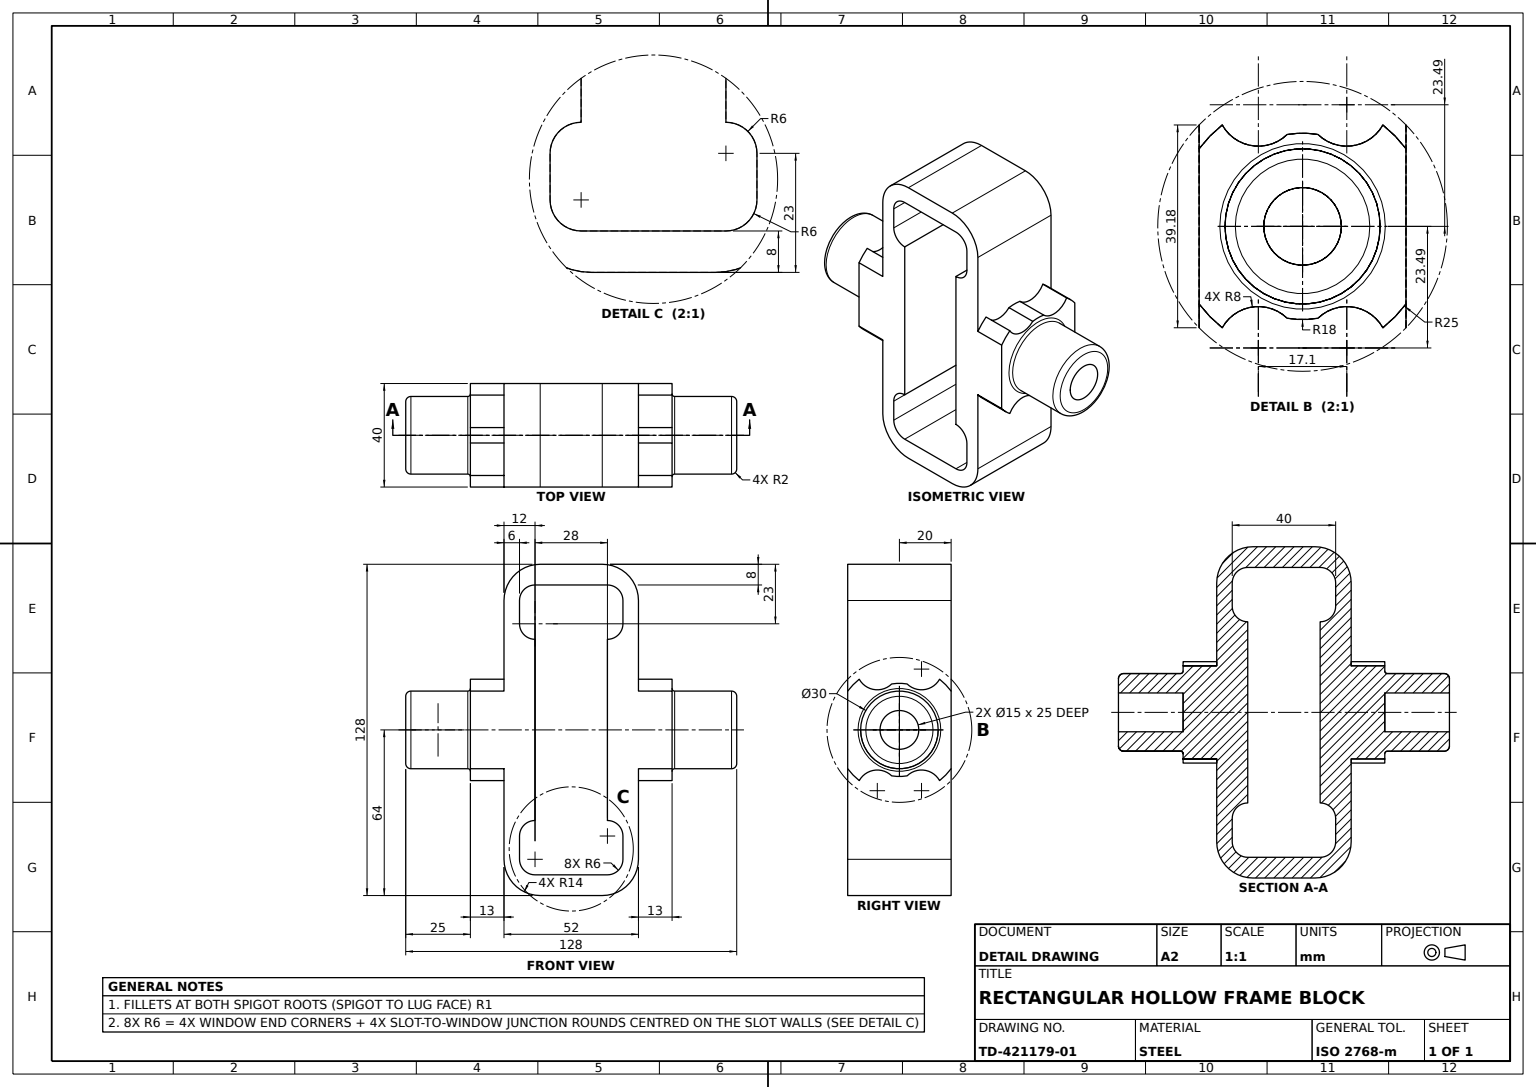
solid
v1 (-64,0,27.5)
v2 (-64,0,12.5)
e1 v1 v2 CIRCLE(AX(P(-64,0,20),D(-1,0,0),D(0,0,1)),7.5)
e2 v2 v1 CIRCLE(AX(P(-64,0,20),D(-1,0,0),D(0,0,1)),7.5)
v3 (-64,0,7)
v4 (-64,0,33)
e3 v3 v4 CIRCLE(AX(P(-64,0,20),D(-1,0,0),D(0,0,1)),13)
e4 v4 v3 CIRCLE(AX(P(-64,0,20),D(-1,0,0),D(0,0,1)),13)
face PLANE(AX(P(-64,0,20),D(-1,0,0),D(0,0,1))) [-e1 -e2] [e3 e4]
v5 (39,-15,40)
v6 (26,-15,40)
e5 v5 v6 LINE
v7 (39,15,40)
e6 v7 v5 LINE
v8 (26,15,40)
e7 v7 v8 LINE
v9 (26,50,40)
e8 v8 v9 LINE
v10 (12,64,40)
e9 v9 v10 CIRCLE(AX(P(12,50,40),D(0,0,1),D(-1,0,0)),14)
v11 (-12,64,40)
e10 v10 v11 LINE
v12 (-26,50,40)
e11 v11 v12 CIRCLE(AX(P(-12,50,40),D(0,0,1),D(-1,0,0)),14)
v13 (-26,15,40)
e12 v12 v13 LINE
v14 (-39,15,40)
e13 v14 v13 LINE
v15 (-39,-15,40)
e14 v15 v14 LINE
v16 (-26,-15,40)
e15 v15 v16 LINE
v17 (-26,-50,40)
e16 v16 v17 LINE
v18 (-12,-64,40)
e17 v17 v18 CIRCLE(AX(P(-12,-50,40),D(0,0,1),D(-1,0,0)),14)
v19 (12,-64,40)
e18 v18 v19 LINE
v20 (26,-50,40)
e19 v19 v20 CIRCLE(AX(P(12,-50,40),D(0,0,1),D(-1,0,0)),14)
e20 v20 v6 LINE
v21 (14,-35,40)
v22 (14,35,40)
e21 v21 v22 LINE
v23 (20,-41,40)
e22 v23 v21 CIRCLE(AX(P(14,-41,40),D(0,0,1),D(-1,0,0)),6)
v24 (20,-50,40)
e23 v24 v23 LINE
v25 (14,-56,40)
e24 v25 v24 CIRCLE(AX(P(14,-50,40),D(0,0,1),D(-1,0,0)),6)
v26 (-14,-56,40)
e25 v26 v25 LINE
v27 (-20,-50,40)
e26 v27 v26 CIRCLE(AX(P(-14,-50,40),D(0,0,1),D(-1,0,0)),6)
v28 (-20,-41,40)
e27 v28 v27 LINE
v29 (-14,-35,40)
e28 v29 v28 CIRCLE(AX(P(-14,-41,40),D(0,0,1),D(-1,0,0)),6)
v30 (-14,35,40)
e29 v30 v29 LINE
v31 (-20,41,40)
e30 v31 v30 CIRCLE(AX(P(-14,41,40),D(0,0,1),D(1,0,0)),6)
v32 (-20,50,40)
e31 v32 v31 LINE
v33 (-14,56,40)
e32 v33 v32 CIRCLE(AX(P(-14,50,40),D(0,0,1),D(-1,0,0)),6)
v34 (14,56,40)
e33 v34 v33 LINE
v35 (20,50,40)
e34 v35 v34 CIRCLE(AX(P(14,50,40),D(0,0,1),D(1,0,0)),6)
v36 (20,41,40)
e35 v36 v35 LINE
e36 v22 v36 CIRCLE(AX(P(14,41,40),D(0,0,1),D(-1,0,0)),6)
face PLANE(AX(P(12,-50,40),D(0,0,-1),D(-1,0,0))) rev [-e5 -e6 e7 e8 e9 e10 e11 e12 -e13 -e14 e15 e16 e17 e18 e19 e20] [-e21 -e22 -e23 -e24 -e25 -e26 -e27 -e28 -e29 -e30 -e31 -e32 -e33 -e34 -e35 -e36]
v37 (20,50,0)
e37 v37 v35 LINE
v38 (20,41,0)
e38 v38 v37 LINE
e39 v38 v36 LINE
face PLANE(AX(P(20,41,0),D(1,0,0),D(0,0,-1))) rev [e35 -e37 -e38 e39]
v39 (40,0,35)
v40 (39,0,36)
e40 v39 v40 CIRCLE(AX(P(40,0,36),D(0,1,0),D(0,0,1)),1)
v41 (40,0,5)
e41 v41 v39 CIRCLE(AX(P(40,0,20),D(1,0,0),D(0,0,-1)),15)
v42 (39,0,4)
e42 v41 v42 CIRCLE(AX(P(40,0,4),D(0,-1,0),D(0,0,-1)),1)
e43 v40 v42 CIRCLE(AX(P(39,0,20),D(-1,0,0),D(0,0,-1)),16)
face TORUS(AX(P(40,0,20),D(1,0,0),D(0,0,-1)),16,1) rev [-e40 -e41 e42 -e43]
v43 (-39,-15,0)
v44 (-26,-15,0)
e44 v43 v44 LINE
v45 (-26,-19.588598,4.46659)
e45 v44 v45 CIRCLE(AX(P(-26,0,20),D(-1,0,0),D(0,0,1)),25)
v46 (-39,-19.588598,4.46659)
e46 v46 v45 LINE
e47 v43 v46 CIRCLE(AX(P(-39,0,20),D(-1,0,0),D(0,0,1)),25)
face CYL(AX(P(-39,0,20),D(1,0,0),D(0,0,-1)),25) [e44 e45 -e46 -e47]
v47 (-14,35,0)
e48 v47 v30 LINE
v48 (-20,41,0)
e49 v48 v47 CIRCLE(AX(P(-14,41,0),D(0,0,1),D(1,0,0)),6)
e50 v48 v31 LINE
face CYL(AX(P(-14,41,0),D(0,0,1),D(1,0,0)),6) rev [-e48 -e49 e50 e30]
v49 (-14,56,0)
e51 v49 v33 LINE
v50 (-20,50,0)
e52 v50 v32 LINE
e53 v49 v50 CIRCLE(AX(P(-14,50,0),D(0,0,1),D(-1,0,0)),6)
face CYL(AX(P(-14,50,0),D(0,0,1),D(1,0,0)),6) rev [e51 e32 -e52 -e53]
v51 (39,-17.751859,17.021494)
v52 (39,-19.588598,4.46659)
e54 v51 v52 CIRCLE(AX(P(39,-23.492316,11.449496),D(-1,0,0),D(0,0,-1)),8)
v53 (26,-17.751859,17.021494)
e55 v51 v53 LINE
v54 (26,-19.588598,4.46659)
e56 v53 v54 CIRCLE(AX(P(26,-23.492316,11.449496),D(-1,0,0),D(0,0,-1)),8)
e57 v52 v54 LINE
face CYL(AX(P(39,-23.492316,11.449496),D(-1,0,0),D(0,0,1)),8) rev [-e54 e55 e56 -e57]
v55 (-39,17.751859,22.978506)
v56 (-26,17.751859,22.978506)
e58 v55 v56 LINE
v57 (-39,19.588598,35.53341)
e59 v57 v55 CIRCLE(AX(P(-39,23.492316,28.550504),D(1,0,0),D(0,0,1)),8)
v58 (-26,19.588598,35.53341)
e60 v57 v58 LINE
e61 v58 v56 CIRCLE(AX(P(-26,23.492316,28.550504),D(1,0,0),D(0,0,1)),8)
face CYL(AX(P(-39,23.492316,28.550504),D(1,0,0),D(0,0,-1)),8) rev [-e58 -e59 e60 e61]
e62 v42 v40 CIRCLE(AX(P(39,0,20),D(-1,0,0),D(0,0,-1)),16)
e63 v39 v41 CIRCLE(AX(P(40,0,20),D(1,0,0),D(0,0,-1)),15)
face TORUS(AX(P(40,0,20),D(1,0,0),D(0,0,-1)),16,1) rev [e40 -e62 -e42 -e63]
v59 (26,50,0)
e64 v9 v59 LINE
v60 (12,64,0)
e65 v59 v60 CIRCLE(AX(P(12,50,0),D(0,0,1),D(-1,0,0)),14)
e66 v10 v60 LINE
face CYL(AX(P(12,50,40),D(0,0,-1),D(-1,0,0)),14) [-e9 e64 e65 -e66]
v61 (39,-17.751859,22.978506)
v62 (26,-17.751859,22.978506)
e67 v61 v62 LINE
v63 (39,-19.588598,35.53341)
e68 v63 v61 CIRCLE(AX(P(39,-23.492316,28.550504),D(-1,0,0),D(0,0,-1)),8)
v64 (26,-19.588598,35.53341)
e69 v63 v64 LINE
e70 v64 v62 CIRCLE(AX(P(26,-23.492316,28.550504),D(-1,0,0),D(0,0,-1)),8)
face CYL(AX(P(39,-23.492316,28.550504),D(-1,0,0),D(0,0,1)),8) rev [-e67 -e68 e69 e70]
v65 (-40,0,35)
v66 (-40,0,5)
e71 v65 v66 CIRCLE(AX(P(-40,0,20),D(-1,0,0),D(0,0,1)),15)
v67 (-62,0,5)
e72 v67 v66 LINE
v68 (-62,0,35)
e73 v67 v68 CIRCLE(AX(P(-62,0,20),D(1,0,0),D(0,0,1)),15)
e74 v68 v65 LINE
face CYL(AX(P(-64,0,20),D(1,0,0),D(0,0,-1)),15) [e71 -e72 e73 e74]
v69 (12,-64,0)
e75 v19 v69 LINE
v70 (26,-50,0)
e76 v69 v70 CIRCLE(AX(P(12,-50,0),D(0,0,1),D(-1,0,0)),14)
e77 v20 v70 LINE
face CYL(AX(P(12,-50,40),D(0,0,-1),D(-1,0,0)),14) [e75 e76 -e77 -e19]
v71 (-12,-64,0)
e78 v18 v71 LINE
v72 (-26,-50,0)
e79 v17 v72 LINE
e80 v72 v71 CIRCLE(AX(P(-12,-50,0),D(0,0,1),D(-1,0,0)),14)
face CYL(AX(P(-12,-50,40),D(0,0,-1),D(-1,0,0)),14) [-e78 -e17 e79 e80]
v73 (39,19.588598,4.46659)
v74 (39,17.751859,17.021494)
e81 v73 v74 CIRCLE(AX(P(39,23.492316,11.449496),D(-1,0,0),D(0,0,-1)),8)
v75 (26,19.588598,4.46659)
e82 v73 v75 LINE
v76 (26,17.751859,17.021494)
e83 v75 v76 CIRCLE(AX(P(26,23.492316,11.449496),D(-1,0,0),D(0,0,-1)),8)
e84 v74 v76 LINE
face CYL(AX(P(39,23.492316,11.449496),D(-1,0,0),D(0,0,1)),8) rev [-e81 e82 e83 -e84]
v77 (26,-15,0)
e85 v54 v77 CIRCLE(AX(P(26,0,20),D(1,0,0),D(0,0,-1)),25)
v78 (39,-15,0)
e86 v78 v77 LINE
e87 v52 v78 CIRCLE(AX(P(39,0,20),D(1,0,0),D(0,0,-1)),25)
face CYL(AX(P(39,0,20),D(-1,0,0),D(0,0,1)),25) [e85 -e86 -e87 e57]
e88 v68 v4 CIRCLE(AX(P(-62,0,33),D(0,-1,0),D(0,0,-1)),2)
e89 v67 v3 CIRCLE(AX(P(-62,0,7),D(0,1,0),D(0,0,1)),2)
face TORUS(AX(P(-62,0,20),D(-1,0,0),D(0,0,1)),13,2) [-e4 -e88 -e73 e89]
e90 v62 v53 CIRCLE(AX(P(26,0,20),D(1,0,0),D(0,0,-1)),18)
e91 v61 v51 CIRCLE(AX(P(39,0,20),D(1,0,0),D(0,0,-1)),18)
face CYL(AX(P(39,0,20),D(-1,0,0),D(0,0,1)),18) [e67 e90 -e55 -e91]
e92 v5 v63 CIRCLE(AX(P(39,0,20),D(1,0,0),D(0,0,-1)),25)
e93 v6 v64 CIRCLE(AX(P(26,0,20),D(1,0,0),D(0,0,-1)),25)
face CYL(AX(P(39,0,20),D(-1,0,0),D(0,0,1)),25) [-e69 -e92 e5 e93]
v79 (-39,0,12.5)
e94 v2 v79 LINE
v80 (-39,0,27.5)
e95 v79 v80 CIRCLE(AX(P(-39,0,20),D(1,0,0),D(0,0,1)),7.5)
e96 v1 v80 LINE
face CYL(AX(P(-64,0,20),D(1,0,0),D(0,0,-1)),7.5) rev [e1 e94 e95 -e96]
v81 (-39,-17.751859,22.978506)
v82 (-39,-19.588598,35.53341)
e97 v81 v82 CIRCLE(AX(P(-39,-23.492316,28.550504),D(1,0,0),D(0,0,1)),8)
v83 (-26,-17.751859,22.978506)
e98 v81 v83 LINE
v84 (-26,-19.588598,35.53341)
e99 v83 v84 CIRCLE(AX(P(-26,-23.492316,28.550504),D(1,0,0),D(0,0,1)),8)
e100 v82 v84 LINE
face CYL(AX(P(-39,-23.492316,28.550504),D(1,0,0),D(0,0,-1)),8) rev [-e97 e98 e99 -e100]
v85 (-20,-41,0)
e101 v85 v28 LINE
v86 (-14,-35,0)
e102 v86 v85 CIRCLE(AX(P(-14,-41,0),D(0,0,1),D(-1,0,0)),6)
e103 v86 v29 LINE
face CYL(AX(P(-14,-41,0),D(0,0,1),D(1,0,0)),6) rev [e28 -e101 -e102 e103]
v87 (-39,0,4)
v88 (-39,0,36)
e104 v87 v88 CIRCLE(AX(P(-39,0,20),D(1,0,0),D(0,0,1)),16)
e105 v88 v87 CIRCLE(AX(P(-39,0,20),D(1,0,0),D(0,0,1)),16)
v89 (-39,17.751859,17.021494)
e106 v55 v89 CIRCLE(AX(P(-39,0,20),D(-1,0,0),D(0,0,1)),18)
v90 (-39,19.588598,4.46659)
e107 v89 v90 CIRCLE(AX(P(-39,23.492316,11.449496),D(1,0,0),D(0,0,1)),8)
v91 (-39,15,0)
e108 v90 v91 CIRCLE(AX(P(-39,0,20),D(-1,0,0),D(0,0,1)),25)
e109 v91 v43 LINE
v92 (-39,-17.751859,17.021494)
e110 v46 v92 CIRCLE(AX(P(-39,-23.492316,11.449496),D(1,0,0),D(0,0,1)),8)
e111 v92 v81 CIRCLE(AX(P(-39,0,20),D(-1,0,0),D(0,0,1)),18)
e112 v82 v15 CIRCLE(AX(P(-39,0,20),D(-1,0,0),D(0,0,1)),25)
e113 v14 v57 CIRCLE(AX(P(-39,0,20),D(-1,0,0),D(0,0,1)),25)
face PLANE(AX(P(-39,0,20),D(-1,0,0),D(0,0,1))) [e104 e105] [e59 e106 e107 e108 e109 e47 e110 e111 e97 e112 e14 e113]
e114 v84 v16 CIRCLE(AX(P(-26,0,20),D(-1,0,0),D(0,0,1)),25)
face CYL(AX(P(-39,0,20),D(1,0,0),D(0,0,-1)),25) [e114 -e15 -e112 e100]
v93 (62,0,35)
e115 v93 v39 LINE
v94 (62,0,5)
e116 v93 v94 CIRCLE(AX(P(62,0,20),D(-1,0,0),D(0,0,-1)),15)
e117 v94 v41 LINE
face CYL(AX(P(64,0,20),D(-1,0,0),D(0,0,1)),15) [e41 -e115 e116 e117]
v95 (14,56,0)
e118 v95 v49 LINE
e119 v95 v34 LINE
face PLANE(AX(P(-14,56,0),D(0,1,0),D(0,0,1))) rev [-e51 -e118 e119 e33]
v96 (14,-35,0)
v97 (14,35,0)
e120 v96 v97 LINE
e121 v96 v21 LINE
e122 v97 v22 LINE
face PLANE(AX(P(14,-35,0),D(1,0,0),D(0,0,-1))) rev [-e120 e121 e21 -e122]
v98 (-20,-50,0)
e123 v85 v98 LINE
e124 v98 v27 LINE
face PLANE(AX(P(-20,-50,0),D(-1,0,0),D(0,-1,0))) rev [-e123 e101 e27 -e124]
e125 v50 v48 LINE
face PLANE(AX(P(-20,41,0),D(-1,0,0),D(0,-1,0))) rev [e31 -e50 -e125 e52]
v99 (-26,17.751859,17.021494)
v100 (-26,19.588598,4.46659)
e126 v99 v100 CIRCLE(AX(P(-26,23.492316,11.449496),D(1,0,0),D(0,0,1)),8)
e127 v90 v100 LINE
e128 v89 v99 LINE
face CYL(AX(P(-39,23.492316,11.449496),D(1,0,0),D(0,0,-1)),8) rev [e126 -e127 -e107 e128]
v101 (64,0,33)
v102 (64,0,7)
e129 v101 v102 CIRCLE(AX(P(64,0,20),D(1,0,0),D(0,0,-1)),13)
e130 v102 v101 CIRCLE(AX(P(64,0,20),D(1,0,0),D(0,0,-1)),13)
v103 (64,0,12.5)
v104 (64,0,27.5)
e131 v103 v104 CIRCLE(AX(P(64,0,20),D(1,0,0),D(0,0,-1)),7.5)
e132 v104 v103 CIRCLE(AX(P(64,0,20),D(1,0,0),D(0,0,-1)),7.5)
face PLANE(AX(P(64,0,20),D(1,0,0),D(0,0,-1))) [e129 e130] [-e131 -e132]
e133 v70 v77 LINE
face PLANE(AX(P(26,-50,40),D(-1,0,0),D(0,0,1))) rev [-e85 -e56 -e90 -e70 -e93 -e20 e77 e133]
v105 (39,0,12.5)
v106 (39,0,27.5)
e134 v105 v106 CIRCLE(AX(P(39,0,20),D(-1,0,0),D(0,0,-1)),7.5)
e135 v106 v105 CIRCLE(AX(P(39,0,20),D(-1,0,0),D(0,0,-1)),7.5)
face PLANE(AX(P(39,0,20),D(1,0,0),D(0,0,-1))) [-e134 -e135]
e136 v94 v93 CIRCLE(AX(P(62,0,20),D(-1,0,0),D(0,0,-1)),15)
face CYL(AX(P(64,0,20),D(-1,0,0),D(0,0,1)),15) [e136 e115 e63 -e117]
v107 (39,19.588598,35.53341)
v108 (26,19.588598,35.53341)
e137 v107 v108 LINE
v109 (39,17.751859,22.978506)
e138 v109 v107 CIRCLE(AX(P(39,23.492316,28.550504),D(-1,0,0),D(0,0,-1)),8)
v110 (26,17.751859,22.978506)
e139 v109 v110 LINE
e140 v110 v108 CIRCLE(AX(P(26,23.492316,28.550504),D(-1,0,0),D(0,0,-1)),8)
face CYL(AX(P(39,23.492316,28.550504),D(-1,0,0),D(0,0,1)),8) rev [-e137 -e138 e139 e140]
v111 (14,-56,0)
e141 v111 v25 LINE
v112 (-14,-56,0)
e142 v112 v111 LINE
e143 v112 v26 LINE
face PLANE(AX(P(-14,-56,0),D(0,-1,0),D(0,0,-1))) rev [-e141 -e142 e143 e25]
e144 v104 v106 LINE
e145 v103 v105 LINE
face CYL(AX(P(64,0,20),D(-1,0,0),D(0,0,1)),7.5) rev [e144 e135 -e145 e131]
v113 (-26,50,0)
v114 (-26,15,0)
e146 v113 v114 LINE
e147 v100 v114 CIRCLE(AX(P(-26,0,20),D(-1,0,0),D(0,0,1)),25)
e148 v56 v99 CIRCLE(AX(P(-26,0,20),D(-1,0,0),D(0,0,1)),18)
e149 v13 v58 CIRCLE(AX(P(-26,0,20),D(-1,0,0),D(0,0,1)),25)
e150 v12 v113 LINE
face PLANE(AX(P(-26,-50,40),D(1,0,0),D(0,0,-1))) rev [e146 -e147 -e126 -e148 -e61 -e149 -e12 e150]
e151 v47 v86 LINE
face PLANE(AX(P(-14,-35,0),D(-1,0,0),D(0,0,1))) rev [e48 e29 -e103 -e151]
e152 v74 v109 CIRCLE(AX(P(39,0,20),D(1,0,0),D(0,0,-1)),18)
e153 v107 v7 CIRCLE(AX(P(39,0,20),D(1,0,0),D(0,0,-1)),25)
v115 (39,15,0)
e154 v78 v115 LINE
e155 v115 v73 CIRCLE(AX(P(39,0,20),D(1,0,0),D(0,0,-1)),25)
face PLANE(AX(P(39,0,20),D(1,0,0),D(0,0,-1))) [e81 e152 e138 e153 e6 e92 e68 e91 e54 e87 e154 e155] [e43 e62]
e156 v71 v69 LINE
face PLANE(AX(P(-12,-64,40),D(0,1,0),D(0,0,1))) rev [-e18 e78 e156 -e75]
v116 (-12,64,0)
e157 v11 v116 LINE
e158 v116 v113 CIRCLE(AX(P(-12,50,0),D(0,0,1),D(-1,0,0)),14)
face CYL(AX(P(-12,50,40),D(0,0,-1),D(-1,0,0)),14) [-e11 e157 e158 -e150]
v117 (20,-50,0)
e159 v117 v24 LINE
v118 (20,-41,0)
e160 v118 v23 LINE
e161 v117 v118 LINE
face PLANE(AX(P(20,-50,0),D(1,0,0),D(0,1,0))) rev [e159 e23 -e160 -e161]
face CYL(AX(P(-39,0,20),D(1,0,0),D(0,0,-1)),25) [e149 -e60 -e113 e13]
e162 v80 v79 CIRCLE(AX(P(-39,0,20),D(1,0,0),D(0,0,1)),7.5)
face PLANE(AX(P(-39,0,20),D(-1,0,0),D(0,0,1))) [-e95 -e162]
e163 v108 v8 CIRCLE(AX(P(26,0,20),D(1,0,0),D(0,0,-1)),25)
e164 v76 v110 CIRCLE(AX(P(26,0,20),D(1,0,0),D(0,0,-1)),18)
v119 (26,15,0)
e165 v119 v75 CIRCLE(AX(P(26,0,20),D(1,0,0),D(0,0,-1)),25)
e166 v119 v59 LINE
face PLANE(AX(P(26,-50,40),D(-1,0,0),D(0,0,1))) rev [-e8 -e163 -e140 -e164 -e83 -e165 e166 -e64]
face CYL(AX(P(39,0,20),D(-1,0,0),D(0,0,1)),25) [-e7 -e153 e137 e163]
face CYL(AX(P(-39,0,20),D(1,0,0),D(0,0,-1)),18) [-e106 e58 e148 -e128]
e167 v111 v117 CIRCLE(AX(P(14,-50,0),D(0,0,1),D(-1,0,0)),6)
face CYL(AX(P(14,-50,0),D(0,0,1),D(1,0,0)),6) rev [e24 -e159 -e167 e141]
e168 v68 v67 CIRCLE(AX(P(-62,0,20),D(1,0,0),D(0,0,1)),15)
face TORUS(AX(P(-62,0,20),D(-1,0,0),D(0,0,1)),13,2) [e88 -e3 -e89 -e168]
e169 v66 v65 CIRCLE(AX(P(-40,0,20),D(-1,0,0),D(0,0,1)),15)
face CYL(AX(P(-64,0,20),D(1,0,0),D(0,0,-1)),15) [e169 -e74 e168 e72]
e170 v115 v119 LINE
face CYL(AX(P(39,0,20),D(-1,0,0),D(0,0,1)),25) [e170 e165 -e82 -e155]
e171 v118 v96 CIRCLE(AX(P(14,-41,0),D(0,0,1),D(-1,0,0)),6)
face CYL(AX(P(14,-41,0),D(0,0,1),D(1,0,0)),6) rev [-e171 e160 e22 -e121]
e172 v97 v38 CIRCLE(AX(P(14,41,0),D(0,0,1),D(-1,0,0)),6)
e173 v37 v95 CIRCLE(AX(P(14,50,0),D(0,0,1),D(1,0,0)),6)
e174 v98 v112 CIRCLE(AX(P(-14,-50,0),D(0,0,1),D(-1,0,0)),6)
e175 v60 v116 LINE
e176 v44 v72 LINE
e177 v91 v114 LINE
face PLANE(AX(P(12,-50,0),D(0,0,-1),D(-1,0,0))) [e161 e171 e120 e172 e38 e173 e118 e53 e125 e49 e151 e102 e123 e174 e142 e167] [-e158 -e175 -e65 -e166 -e170 -e154 e86 -e133 -e76 -e156 -e80 -e176 -e44 -e109 e177 -e146]
v120 (-26,-17.751859,17.021494)
e178 v45 v120 CIRCLE(AX(P(-26,-23.492316,11.449496),D(1,0,0),D(0,0,1)),8)
e179 v92 v120 LINE
face CYL(AX(P(-39,-23.492316,11.449496),D(1,0,0),D(0,0,-1)),8) rev [-e110 e46 e178 -e179]
face CYL(AX(P(64,0,20),D(-1,0,0),D(0,0,1)),7.5) rev [-e144 e132 e145 e134]
e180 v65 v88 CIRCLE(AX(P(-40,0,36),D(0,-1,0),D(0,0,-1)),1)
e181 v66 v87 CIRCLE(AX(P(-40,0,4),D(0,1,0),D(0,0,1)),1)
face TORUS(AX(P(-40,0,20),D(-1,0,0),D(0,0,1)),16,1) rev [-e71 e180 -e104 -e181]
face CYL(AX(P(14,41,0),D(0,0,1),D(1,0,0)),6) rev [e122 e36 -e39 -e172]
e182 v94 v102 CIRCLE(AX(P(62,0,7),D(0,-1,0),D(0,0,-1)),2)
e183 v93 v101 CIRCLE(AX(P(62,0,33),D(0,1,0),D(0,0,1)),2)
face TORUS(AX(P(62,0,20),D(1,0,0),D(0,0,-1)),13,2) [-e130 -e182 -e116 e183]
face CYL(AX(P(39,0,20),D(-1,0,0),D(0,0,1)),18) [e84 e164 -e139 -e152]
face CYL(AX(P(14,50,0),D(0,0,1),D(1,0,0)),6) rev [-e119 -e173 e37 e34]
e184 v120 v83 CIRCLE(AX(P(-26,0,20),D(-1,0,0),D(0,0,1)),18)
face CYL(AX(P(-39,0,20),D(1,0,0),D(0,0,-1)),18) [-e98 -e111 e179 e184]
face CYL(AX(P(-14,-50,0),D(0,0,1),D(1,0,0)),6) rev [e124 e26 -e143 -e174]
face TORUS(AX(P(62,0,20),D(1,0,0),D(0,0,-1)),13,2) [e182 -e129 -e183 -e136]
face TORUS(AX(P(-40,0,20),D(-1,0,0),D(0,0,1)),16,1) rev [-e180 -e169 e181 -e105]
face CYL(AX(P(-64,0,20),D(1,0,0),D(0,0,-1)),7.5) rev [e162 -e94 e2 e96]
face PLANE(AX(P(-12,64,40),D(0,-1,0),D(0,0,-1))) rev [e175 -e157 -e10 e66]
face PLANE(AX(P(-26,-50,40),D(1,0,0),D(0,0,-1))) rev [-e45 e176 -e79 -e16 -e114 -e99 -e184 -e178]
face CYL(AX(P(-39,0,20),D(1,0,0),D(0,0,-1)),25) [e147 -e177 -e108 e127]
